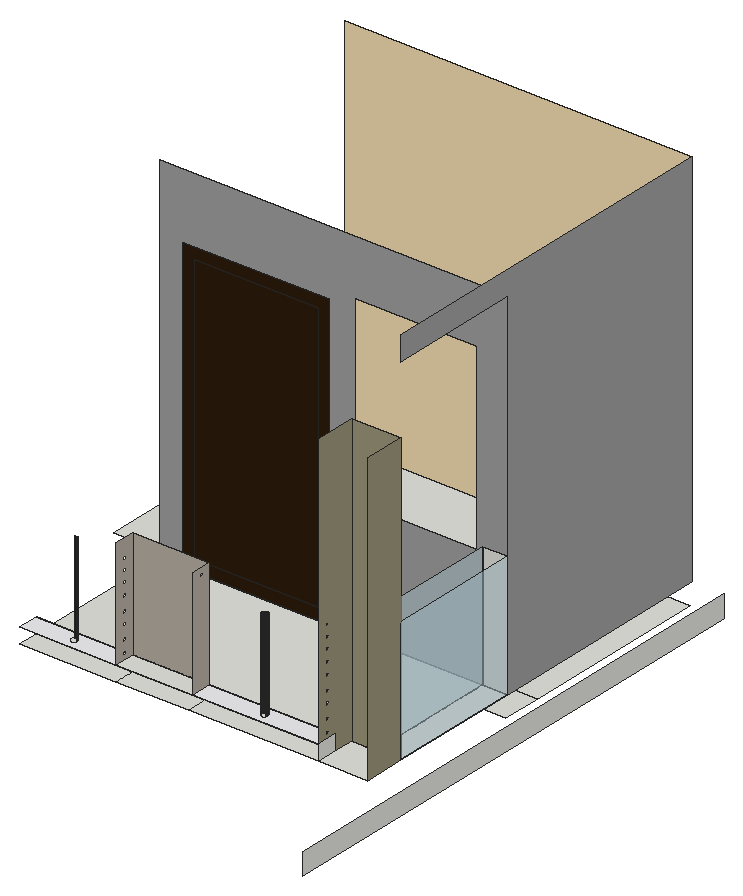
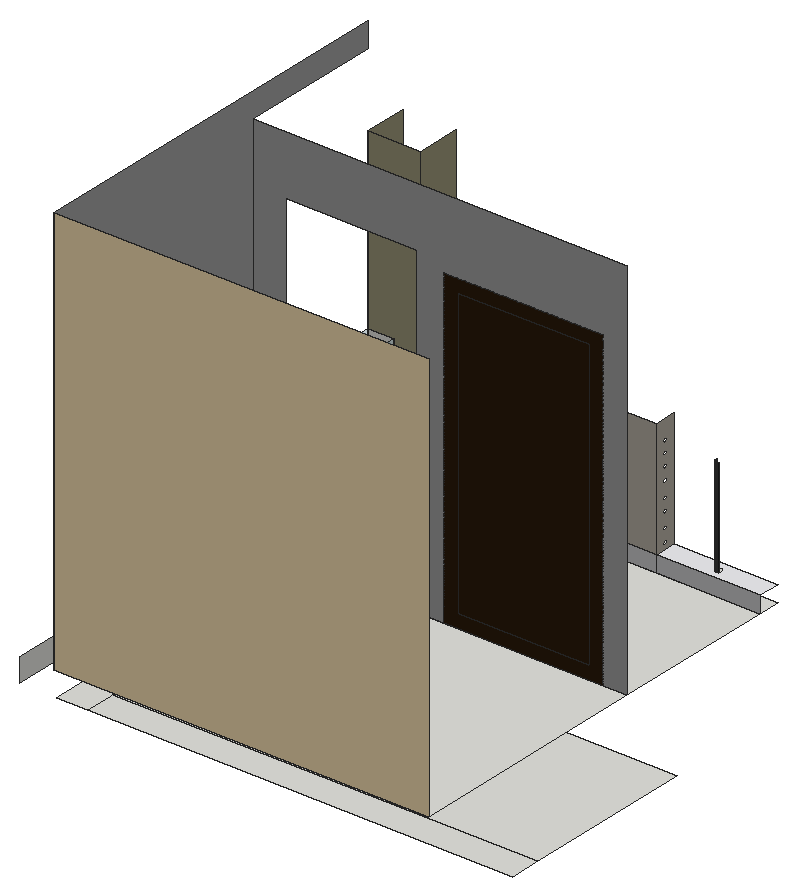
# SketchUp Ruby script. Lengths in inches.
U = 1.inch
M = Sketchup.active_model
def pt(a) = Geom::Point3d.new(a.map { |v| v * U })
def face(e, loops, mat)
  f = e.add_face(loops[0].map { |a| pt(a) })
  loops[1..].each { |l| e.add_face(l.map { |a| pt(a) }).erase! }
  f.material = f.back_material = mat if mat
  f
end
# faces: each face lists its corners as indices into pts; further lists are holes
def faces(e, pts, list, mat = nil) = list.each { |f| face(e, (f[0].is_a?(Array) ? f : [f]).map { |l| l.map { |i| pts[i] } }, mat) }
# xy, xz, yz: faces in a plane at the given z, y or x. An outline is a flat list of corners, or four numbers for a rectangle; further outlines are holes
def ring(l) = l.size == 4 ? [[l[0], l[1]], [l[2], l[1]], [l[2], l[3]], [l[0], l[3]]] : l.each_slice(2).to_a
def flat(e, list, mat, &to3) = list.each { |f| face(e, (f[0].is_a?(Array) ? f : [f]).map { |l| ring(l).map { |u, v| to3.(u, v) } }, mat) }
def xy(e, z, list, mat = nil) = flat(e, list, mat) { |x, y| [x, y, z] }
def xz(e, y, list, mat = nil) = flat(e, list, mat) { |x, z| [x, y, z] }
def yz(e, x, list, mat = nil) = flat(e, list, mat) { |y, z| [x, y, z] }
def lines(e, pts, list) = list.each { |a, b| e.add_line(pt(pts[a]), pt(pts[b])) }
# prism: a flat outline (further loops are holes) pulled along v
def prism(e, loops, v, mat = nil)
  f = face(e, loops, mat); d = Geom::Vector3d.new(v.map { |x| x * U })
  f.pushpull(f.normal.samedirection?(d) ? d.length : -d.length)
end
def box(e, o, s, mat = nil) = prism(e, [[o, [o[0] + s[0], o[1], o[2]], [o[0] + s[0], o[1] + s[1], o[2]], [o[0], o[1] + s[1], o[2]]]], [0, 0, s[2]], mat)
def at(x, y, z, deg = 0) = Geom::Transformation.translation(pt([x, y, z])) * Geom::Transformation.rotation(ORIGIN, Z_AXIS, deg.degrees)
def axes(o, x, y, z) = Geom::Transformation.new([*x, 0, *y, 0, *z, 0, *pt(o).to_a, 1])
def part(name) = M.definitions.add(name)
# library, detail: a bought-in or finely detailed component or shape, given as its bounding box
def library(name, o, s) = part(name).tap { |d| box(d.entities, o, s) }
def detail(e, o, s) = box(e.add_group.entities, o, s)
def put(e, d, t, mat = nil) = e.add_instance(d, t).tap { |i| i.material = mat if mat }
def group(e, t, mat = nil) = e.add_group.tap { |g| g.transformation = t; g.material = mat if mat }.entities
root = M.entities
M.materials.add("[0034_Wheat]").color = [245, 222, 179]
M.materials.add("[0136_Charcoal]").color = [35, 35, 35]
M.materials.add("[Blinds Vertical Pattern]1").color = [239, 239, 242]
M.materials.add("[Blinds Vertical Stripe Gray]2").color = [160, 160, 160]
M.materials.add("[Polished Concrete New]").color = [200, 200, 203]
M.materials.add("[Stone Coursed Rough]").color = [155, 150, 122]
M.materials.add("[Stone Masonry Multi]").color = [182, 175, 164]
M.materials.add("[Translucent Glass Safety]").color = [204, 235, 244]
M.materials["[Translucent Glass Safety]"].alpha = 0.5
M.materials.add("[Wood Floor Parquet]").color = [45, 28, 12]
xy(root,130.875,[[277.86,280.61,297.85,292.92],[164.37,292.92,164.37,343.79,288.72,343.79,288.72,352.92,297.85,352.92,297.85,292.92],[164.37,343.79,288.72,352.92]])
xy(root,137.875,[[189.02,225.17,219.28,231.66],[219.28,225.17,242.08,231.66],[242.08,225.17,283.04,231.66],[283.04,225.17,298.6,238.17],[189.02,231.66,283.04,231.66,283.04,238.17,290.82,238.17,290.82,280.2,189.02,280.2],
  [290.82,238.17,298.6,280.2],[189.02,280.2,298.6,352.92]])
xy(root,142.6875,[[219.28,225.17,243.46,231.66],[203.52,227.49,203.28,227.52,203.05,227.61,202.86,227.76,202.71,227.96,202.61,228.18,202.58,228.42,202.61,228.67,202.71,228.89,202.86,229.09,203.05,229.24,203.28,229.33,203.52,229.36,203.76,229.33,203.99,229.24,204.18,229.09,204.33,228.89,204.43,228.67,204.46,228.42,204.43,228.18,204.33,227.96,204.18,227.76,203.99,227.61,203.76,227.52],[263.52,227.49,263.28,227.52,263.05,227.61,262.86,227.76,262.71,227.96,262.61,228.18,262.58,228.42,262.61,228.67,262.71,228.89,262.86,229.09,263.05,229.24,263.28,229.33,263.52,229.36,263.76,229.33,263.99,229.24,264.18,229.09,264.33,228.89,264.43,228.67,264.46,228.42,264.43,228.18,264.33,227.96,264.18,227.76,263.99,227.61,263.76,227.52]])
xy(root,142.6875,[[[189.02,225.17,219.28,231.66],[203.52,227.49,203.28,227.52,203.05,227.61,202.86,227.76,202.71,227.96,202.61,228.18,202.58,228.42,202.61,228.67,202.71,228.89,202.86,229.09,203.05,229.24,203.28,229.33,203.52,229.36,203.76,229.33,203.99,229.24,204.18,229.09,204.33,228.89,204.43,228.67,204.46,228.42,204.43,228.18,204.33,227.96,204.18,227.76,203.99,227.61,203.76,227.52]],[[243.46,225.17,283.04,231.66],[263.52,227.49,263.28,227.52,263.05,227.61,262.86,227.76,262.71,227.96,262.61,228.18,262.58,228.42,262.61,228.67,262.71,228.89,262.86,229.09,263.05,229.24,263.28,229.33,263.52,229.36,263.76,229.33,263.99,229.24,264.18,229.09,264.33,228.89,264.43,228.67,264.46,228.42,264.43,228.18,264.33,227.96,264.18,227.76,263.99,227.61,263.76,227.52]]],"[Blinds Vertical Pattern]1")
xz(root,231.66,[[189.02,137.875,219.28,142.6875],[219.28,137.875,242.08,142.6875],[242.08,137.875,283.04,142.6875]],"[Polished Concrete New]")
xz(root,231.66,[[219.28,142.6875,243.46,177]],"[Stone Masonry Multi]")
xz(root,238.17,[[290.82,137.875,298.6,177]])
xz(root,238.17,[[283.04,137.875,283.04,228.8125,298.6,228.8125,298.6,177,290.82,177,290.82,137.875]],"[Stone Coursed Rough]")
xz(root,280.2,[[290.82,137.875,298.6,177]])
xz(root,280.2,[[[189.02,137.875,196.1,137.875,196.1,229.875,242.6,229.875,242.6,137.875,290.82,137.875,290.82,177,298.6,177,298.6,250.375,189.02,250.375],[250.45,175.375,289.08,233.0625]]],"[Blinds Vertical Stripe Gray]2")
xz(root,280.2,[[[196.1,137.875,242.6,229.875],[200,141.77,238.71,225.98]],[200,141.77,238.71,225.98]],"[Wood Floor Parquet]")
xz(root,352.92,[[189.02,137.875,298.6,257.875]],"[0034_Wheat]")
yz(root,219.28,[[[225.17,142.6875,231.66,177],[228.53,170.81,228.6875,170.83,228.84,170.89,228.97,170.99,229.07,171.12,229.13,171.27,229.15,171.43,229.13,171.59,229.07,171.74,228.97,171.875,228.84,171.97,228.6875,172.04,228.53,172.06,228.36,172.04,228.21,171.97,228.08,171.875,227.98,171.74,227.92,171.59,227.9,171.43,227.92,171.27,227.98,171.12,228.08,170.99,228.21,170.89,228.36,170.83],[228.53,147.74,228.6875,147.77,228.84,147.83,228.97,147.93,229.07,148.06,229.13,148.21,229.15,148.37,229.13,148.53,229.07,148.68,228.97,148.8125,228.84,148.91,228.6875,148.97,228.53,148.99,228.36,148.97,228.21,148.91,228.08,148.8125,227.98,148.68,227.92,148.53,227.9,148.37,227.92,148.21,227.98,148.06,228.08,147.93,228.21,147.83,228.36,147.77],[228.53,167.43,228.6875,167.45,228.84,167.52,228.97,167.62,229.07,167.74,229.13,167.9,229.15,168.06,229.13,168.22,229.07,168.37,228.97,168.5,228.84,168.6,228.6875,168.66,228.53,168.68,228.36,168.66,228.21,168.6,228.08,168.5,227.98,168.37,227.92,168.22,227.9,168.06,227.92,167.9,227.98,167.74,228.08,167.62,228.21,167.52,228.36,167.45],[228.53,152.12,228.6875,152.14,228.84,152.2,228.97,152.3,229.07,152.43,229.13,152.58,229.15,152.74,229.13,152.91,229.07,153.06,228.97,153.1875,228.84,153.29,228.6875,153.35,228.53,153.37,228.36,153.35,228.21,153.29,228.08,153.1875,227.98,153.06,227.92,152.91,227.9,152.74,227.92,152.58,227.98,152.43,228.08,152.3,228.21,152.2,228.36,152.14],[228.53,163.93,228.6875,163.95,228.84,164.02,228.97,164.12,229.07,164.24,229.13,164.4,229.15,164.56,229.13,164.72,229.07,164.87,228.97,165,228.84,165.1,228.6875,165.16,228.53,165.18,228.36,165.16,228.21,165.1,228.08,165,227.98,164.87,227.92,164.72,227.9,164.56,227.92,164.4,227.98,164.24,228.08,164.12,228.21,164.02,228.36,163.95],[228.53,155.62,228.6875,155.64,228.84,155.7,228.97,155.8,229.07,155.93,229.13,156.08,229.15,156.24,229.13,156.41,229.07,156.56,228.97,156.6875,228.84,156.79,228.6875,156.85,228.53,156.87,228.36,156.85,228.21,156.79,228.08,156.6875,227.98,156.56,227.92,156.41,227.9,156.24,227.92,156.08,227.98,155.93,228.08,155.8,228.21,155.7,228.36,155.64],[228.53,160.18,228.6875,160.2,228.84,160.27,228.97,160.37,229.07,160.49,229.13,160.65,229.15,160.81,229.13,160.97,229.07,161.12,228.97,161.25,228.84,161.35,228.6875,161.41,228.53,161.43,228.36,161.41,228.21,161.35,228.08,161.25,227.98,161.12,227.92,160.97,227.9,160.81,227.92,160.65,227.98,160.49,228.08,160.37,228.21,160.27,228.36,160.2],[228.53,143.87,228.6875,143.89,228.84,143.95,228.97,144.05,229.07,144.18,229.13,144.33,229.15,144.49,229.13,144.66,229.07,144.81,228.97,144.9375,228.84,145.04,228.6875,145.1,228.53,145.12,228.36,145.1,228.21,145.04,228.08,144.9375,227.98,144.81,227.92,144.66,227.9,144.49,227.92,144.33,227.98,144.18,228.08,144.05,228.21,143.95,228.36,143.89]]],"[Stone Masonry Multi]")
yz(root,243.46,[[[225.17,142.6875,231.66,177],[228.44,174.54,228.3,174.5625,228.16,174.62,228.04,174.71,227.95,174.83,227.9,174.96,227.88,175.11,227.9,175.25,227.95,175.39,228.04,175.5,228.16,175.59,228.3,175.65,228.44,175.67,228.59,175.65,228.72,175.59,228.84,175.5,228.93,175.39,228.98,175.25,229,175.11,228.98,174.96,228.93,174.83,228.84,174.71,228.72,174.62,228.59,174.5625]]],"[Stone Masonry Multi]")
yz(root,283.04,[[225.17,137.875,231.66,142.6875]])
yz(root,283.04,[[[231.66,137.875,231.66,142.6875,225.17,142.6875,225.17,228.8125,238.17,228.8125,238.17,137.875],[228.53,170.81,228.6875,170.83,228.84,170.89,228.97,170.99,229.07,171.12,229.13,171.27,229.15,171.43,229.13,171.59,229.07,171.74,228.97,171.875,228.84,171.97,228.6875,172.04,228.53,172.06,228.36,172.04,228.21,171.97,228.08,171.875,227.98,171.74,227.92,171.59,227.9,171.43,227.92,171.27,227.98,171.12,228.08,170.99,228.21,170.89,228.36,170.83],[228.53,167.43,228.6875,167.45,228.84,167.52,228.97,167.62,229.07,167.74,229.13,167.9,229.15,168.06,229.13,168.22,229.07,168.37,228.97,168.5,228.84,168.6,228.6875,168.66,228.53,168.68,228.36,168.66,228.21,168.6,228.08,168.5,227.98,168.37,227.92,168.22,227.9,168.06,227.92,167.9,227.98,167.74,228.08,167.62,228.21,167.52,228.36,167.45],[228.53,163.93,228.6875,163.95,228.84,164.02,228.97,164.12,229.07,164.24,229.13,164.4,229.15,164.56,229.13,164.72,229.07,164.87,228.97,165,228.84,165.1,228.6875,165.16,228.53,165.18,228.36,165.16,228.21,165.1,228.08,165,227.98,164.87,227.92,164.72,227.9,164.56,227.92,164.4,227.98,164.24,228.08,164.12,228.21,164.02,228.36,163.95],[228.53,160.18,228.6875,160.2,228.84,160.27,228.97,160.37,229.07,160.49,229.13,160.65,229.15,160.81,229.13,160.97,229.07,161.12,228.97,161.25,228.84,161.35,228.6875,161.41,228.53,161.43,228.36,161.41,228.21,161.35,228.08,161.25,227.98,161.12,227.92,160.97,227.9,160.81,227.92,160.65,227.98,160.49,228.08,160.37,228.21,160.27,228.36,160.2],[228.53,155.62,228.6875,155.64,228.84,155.7,228.97,155.8,229.07,155.93,229.13,156.08,229.15,156.24,229.13,156.41,229.07,156.56,228.97,156.6875,228.84,156.79,228.6875,156.85,228.53,156.87,228.36,156.85,228.21,156.79,228.08,156.6875,227.98,156.56,227.92,156.41,227.9,156.24,227.92,156.08,227.98,155.93,228.08,155.8,228.21,155.7,228.36,155.64],[228.53,152.12,228.6875,152.14,228.84,152.2,228.97,152.3,229.07,152.43,229.13,152.58,229.15,152.74,229.13,152.91,229.07,153.06,228.97,153.1875,228.84,153.29,228.6875,153.35,228.53,153.37,228.36,153.35,228.21,153.29,228.08,153.1875,227.98,153.06,227.92,152.91,227.9,152.74,227.92,152.58,227.98,152.43,228.08,152.3,228.21,152.2,228.36,152.14],[228.53,147.74,228.6875,147.77,228.84,147.83,228.97,147.93,229.07,148.06,229.13,148.21,229.15,148.37,229.13,148.53,229.07,148.68,228.97,148.8125,228.84,148.91,228.6875,148.97,228.53,148.99,228.36,148.97,228.21,148.91,228.08,148.8125,227.98,148.68,227.92,148.53,227.9,148.37,227.92,148.21,227.98,148.06,228.08,147.93,228.21,147.83,228.36,147.77],[228.53,143.87,228.6875,143.89,228.84,143.95,228.97,144.05,229.07,144.18,229.13,144.33,229.15,144.49,229.13,144.66,229.07,144.81,228.97,144.9375,228.84,145.04,228.6875,145.1,228.53,145.12,228.36,145.1,228.21,145.04,228.08,144.9375,227.98,144.81,227.92,144.66,227.9,144.49,227.92,144.33,227.98,144.18,228.08,144.05,228.21,143.95,228.36,143.89],[228.44,174.54,228.59,174.5625,228.72,174.62,228.84,174.71,228.93,174.83,228.98,174.96,229,175.11,228.98,175.25,228.93,175.39,228.84,175.5,228.72,175.59,228.59,175.65,228.44,175.67,228.3,175.65,228.16,175.59,228.04,175.5,227.95,175.39,227.9,175.25,227.88,175.11,227.9,174.96,227.95,174.83,228.04,174.71,228.16,174.62,228.3,174.5625]]],"[Stone Coursed Rough]")
yz(root,290.82,[[238.17,137.875,280.2,177]],"[Translucent Glass Safety]")
yz(root,298.6,[[280.2,137.875,352.92,137.875,352.92,257.875,238.17,257.875,238.17,250.375,280.2,250.375]],"[Blinds Vertical Stripe Gray]2")
yz(root,298.6,[[225.17,137.875,238.17,228.8125]],"[Stone Coursed Rough]")
yz(root,298.6,[[238.17,137.875,280.2,177]],"[Translucent Glass Safety]")
yz(root,308.53,[[187.36,130.875,352.92,137.875]])
p = [[262.61,228.18,142.6875],[262.71,227.96,142.6875],[262.71,227.96,171.3125],[262.61,228.18,171.3125],[264.33,227.96,142.6875],[264.43,228.18,142.6875],
  [264.43,228.18,171.3125],[264.33,227.96,171.3125],[204.43,228.18,142.6875],[204.46,228.42,142.6875],[204.46,228.42,171.43],[204.43,228.18,171.43],
  [262.58,228.42,142.6875],[262.58,228.42,171.3125],[264.46,228.42,142.6875],[264.46,228.42,171.3125],[204.43,228.67,142.6875],[204.43,228.67,171.43],
  [262.61,228.67,142.6875],[262.61,228.67,171.3125],[264.43,228.67,142.6875],[264.43,228.67,171.3125],[204.33,228.89,142.6875],[204.33,228.89,171.43],
  [262.71,228.89,142.6875],[262.71,228.89,171.3125],[264.33,228.89,142.6875],[264.33,228.89,171.3125],[204.18,229.09,142.6875],[204.18,229.09,171.43],
  [262.86,229.09,142.6875],[262.86,229.09,171.3125],[264.18,229.09,142.6875],[264.18,229.09,171.3125],[203.99,229.24,142.6875],[203.99,229.24,171.43],
  [204.1,229.15,171.43],[263.05,229.24,142.6875],[263.05,229.24,171.3125],[263.99,229.24,142.6875],[263.99,229.24,171.3125],[203.28,229.33,142.6875],
  [203.05,229.24,142.6875],[203.05,229.24,171.43],[203.28,229.33,171.43],[203.76,229.33,142.6875],[203.76,229.33,171.43],[263.28,229.33,142.6875],
  [263.28,229.33,171.3125],[263.76,229.33,142.6875],[263.76,229.33,171.3125],[203.52,229.36,142.6875],[203.52,229.36,171.43],[263.52,229.36,142.6875],
  [263.52,229.36,171.3125]]
faces(root,p,[[0,1,2,3],[4,5,6,7],[8,9,10,11],[12,0,3,13],[5,14,15,6],[9,16,17,10],[18,12,13,19],[14,20,21,15],
  [16,22,23,17],[24,18,19,25],[20,26,27,21],[22,28,29,23],[30,24,25,31],[26,32,33,27],[28,34,35,36,29],[37,30,31,38],
  [32,39,40,33],[41,42,43,44],[34,45,46,35],[47,37,38,48],[39,49,50,40],[51,41,44,52],[45,51,52,46],[53,47,48,54],
  [49,53,54,50]],"[0136_Charcoal]")
